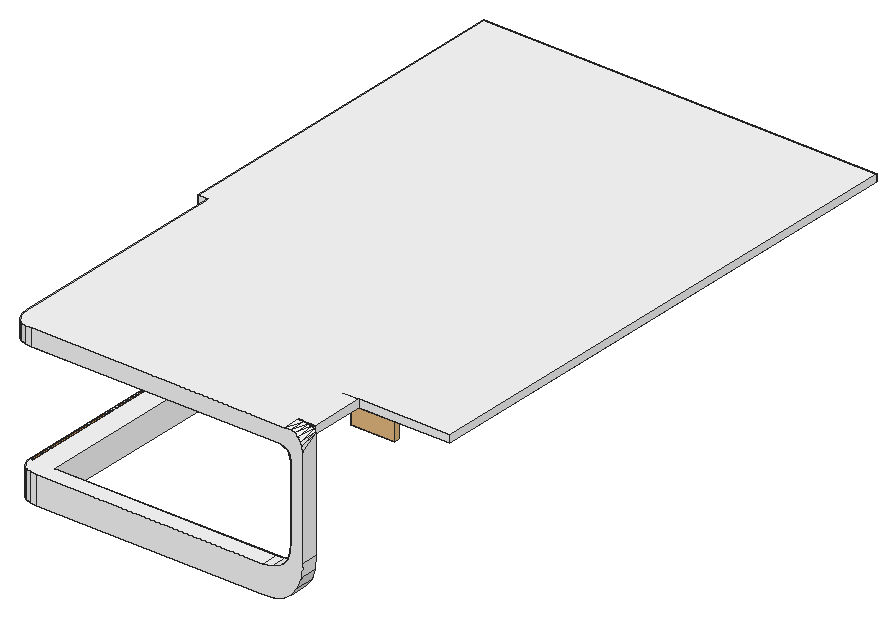
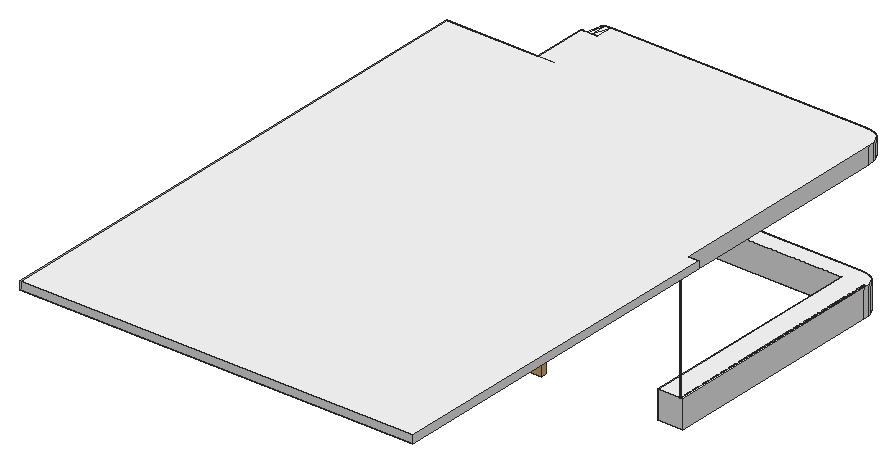
# SketchUp Ruby script. Lengths in inches.
U = 1.inch
M = Sketchup.active_model
def pt(a) = Geom::Point3d.new(a.map { |v| v * U })
def face(e, loops, mat)
  f = e.add_face(loops[0].map { |a| pt(a) })
  loops[1..].each { |l| e.add_face(l.map { |a| pt(a) }).erase! }
  f.material = f.back_material = mat if mat
  f
end
# faces: each face lists its corners as indices into pts; further lists are holes
def faces(e, pts, list, mat = nil) = list.each { |f| face(e, (f[0].is_a?(Array) ? f : [f]).map { |l| l.map { |i| pts[i] } }, mat) }
# xy, xz, yz: faces in a plane at the given z, y or x. An outline is a flat list of corners, or four numbers for a rectangle; further outlines are holes
def ring(l) = l.size == 4 ? [[l[0], l[1]], [l[2], l[1]], [l[2], l[3]], [l[0], l[3]]] : l.each_slice(2).to_a
def flat(e, list, mat, &to3) = list.each { |f| face(e, (f[0].is_a?(Array) ? f : [f]).map { |l| ring(l).map { |u, v| to3.(u, v) } }, mat) }
def xy(e, z, list, mat = nil) = flat(e, list, mat) { |x, y| [x, y, z] }
def xz(e, y, list, mat = nil) = flat(e, list, mat) { |x, z| [x, y, z] }
def yz(e, x, list, mat = nil) = flat(e, list, mat) { |y, z| [x, y, z] }
def lines(e, pts, list) = list.each { |a, b| e.add_line(pt(pts[a]), pt(pts[b])) }
# prism: a flat outline (further loops are holes) pulled along v
def prism(e, loops, v, mat = nil)
  f = face(e, loops, mat); d = Geom::Vector3d.new(v.map { |x| x * U })
  f.pushpull(f.normal.samedirection?(d) ? d.length : -d.length)
end
def box(e, o, s, mat = nil) = prism(e, [[o, [o[0] + s[0], o[1], o[2]], [o[0] + s[0], o[1] + s[1], o[2]], [o[0], o[1] + s[1], o[2]]]], [0, 0, s[2]], mat)
def at(x, y, z, deg = 0) = Geom::Transformation.translation(pt([x, y, z])) * Geom::Transformation.rotation(ORIGIN, Z_AXIS, deg.degrees)
def axes(o, x, y, z) = Geom::Transformation.new([*x, 0, *y, 0, *z, 0, *pt(o).to_a, 1])
def part(name) = M.definitions.add(name)
# library, detail: a bought-in or finely detailed component or shape, given as its bounding box
def library(name, o, s) = part(name).tap { |d| box(d.entities, o, s) }
def detail(e, o, s) = box(e.add_group.entities, o, s)
def put(e, d, t, mat = nil) = e.add_instance(d, t).tap { |i| i.material = mat if mat }
def group(e, t, mat = nil) = e.add_group.tap { |g| g.transformation = t; g.material = mat if mat }.entities
root = M.entities
M.materials.add("1056 AP 9903 Mellow Melon-N").color = [219, 142, 59]
M.materials.add("1117 AP 9945 Muted Auburn-N").color = [162, 88, 63]
M.materials.add("CTS CNC Default").color = [255, 255, 255]
c1 = library("Untitled",[0,0,0],[36,4.39,84])
c2 = part("Recessed ceiling light")
xy(c2.entities,-1,[[6,2,7.04,2.14,8,2.54,8.83,3.17,9.46,4,9.86,4.96,10,6,9.86,7.04,9.46,8,8.83,8.83,8,9.46,7.04,9.86,6,10,4.96,9.86,4,9.46,3.17,8.83,2.54,8,2.14,7.04,2,6,2.14,4.96,2.54,4,3.17,3.17,4,2.54,4.96,2.14]],"1117 AP 9945 Muted Auburn-N")
xy(c2.entities,0,[[[6,0,7.55,0.2,9,0.8,10.24,1.76,11.2,3,11.8,4.45,12,6,11.8,7.55,11.2,9,10.24,10.24,9,11.2,7.55,11.8,6,12,4.45,11.8,3,11.2,1.76,10.24,0.8,9,0.2,7.55,0,6,0.2,4.45,0.8,3,1.76,1.76,3,0.8,4.45,0.2],[6,2,4.96,2.14,4,2.54,3.17,3.17,2.54,4,2.14,4.96,2,6,2.14,7.04,2.54,8,3.17,8.83,4,9.46,4.96,9.86,6,10,7.04,9.86,8,9.46,8.83,8.83,9.46,8,9.86,7.04,10,6,9.86,4.96,9.46,4,8.83,3.17,8,2.54,7.04,2.14]]],"1117 AP 9945 Muted Auburn-N")
p = [[4.96,2.14,0],[6,2,0],[6,2,-1],[4.96,2.14,-1],[7.04,2.14,0],[7.04,2.14,-1],
  [4,2.54,0],[4,2.54,-1],[8,2.54,0],[8,2.54,-1],[3.17,3.17,0],[3.17,3.17,-1],
  [8.83,3.17,0],[8.83,3.17,-1],[2.54,4,0],[2.54,4,-1],[9.46,4,0],[9.46,4,-1],
  [2.14,4.96,0],[2.14,4.96,-1],[9.86,4.96,0],[9.86,4.96,-1],[2,6,0],[2,6,-1],
  [10,6,0],[10,6,-1],[2.14,7.04,0],[2.14,7.04,-1],[9.86,7.04,0],[9.86,7.04,-1],
  [2.54,8,0],[2.54,8,-1],[9.46,8,0],[9.46,8,-1],[3.17,8.83,0],[3.17,8.83,-1],
  [8.83,8.83,0],[8.83,8.83,-1],[4,9.46,0],[4,9.46,-1],[8,9.46,0],[8,9.46,-1],
  [4.96,9.86,0],[4.96,9.86,-1],[7.04,9.86,0],[7.04,9.86,-1],[6,10,0],[6,10,-1]]
faces(c2.entities,p,[[0,1,2,3],[1,4,5,2],[6,0,3,7],[4,8,9,5],[10,6,7,11],[8,12,13,9],[14,10,11,15],[12,16,17,13],
  [18,14,15,19],[16,20,21,17],[22,18,19,23],[20,24,25,21],[26,22,23,27],[24,28,29,25],[30,26,27,31],[28,32,33,29],
  [34,30,31,35],[32,36,37,33],[38,34,35,39],[36,40,41,37],[42,38,39,43],[40,44,45,41],[46,42,43,47],[44,46,47,45]],"1117 AP 9945 Muted Auburn-N")
xy(root,145.75,[[14.35,13.79,15.0625,202.3125]],"1056 AP 9903 Mellow Melon-N")
xz(root,202.3125,[[14.35,145.75,15.0625,238.4375]],"1056 AP 9903 Mellow Melon-N")
p = [[15.0625,202.3125,145.75],[15.0625,202.3125,238.4375],[15.0625,13.79,145.75]]
lines(root,p,[[0,1],[2,0]])
put(root,c1,at(123.5625,204.4,126))
g1 = group(root,at(21.875,58.1875,246),"CTS CNC Default")
xy(g1,-123,[[7.7,-58.1875,2.53,-57.72,-1.69,-56.31,-4.98,-53.96,-7.33,-50.67,-8.74,-46.45,-9.21,-41.28,-9.21,144.125,11.625,144.125,11.625,-44.375,191.93,-44.375,191.93,-58.1875]])
xy(g1,-100.25,[[7.7,-58.1875,193.39,-58.1875,193.39,-44.375,11.625,-44.375,11.625,144.125,-9.21,144.125,-9.21,-41.28,-8.74,-46.45,-7.33,-50.67,-4.98,-53.96,-1.69,-56.31,2.53,-57.72]])
xy(g1,-7.5625,[[4.05,-58.1875,-1.35,-57.7,-5.77,-56.22,-9.21,-53.77,-11.66,-50.33,-13.13,-45.91,-13.625,-40.51,-13.625,144.125,0,144.125,0,-44.375,205.85,-44.375,205.85,-58.1875]])
xy(g1,0,[[0,-44.375,0,144.125,300,144.125,300,0,225.17,0,225.17,-44.375]],"1117 AP 9945 Muted Auburn-N")
xy(g1,0,[[-21.875,144.125,300,436.5]],"CTS CNC Default")
xy(g1,6,[[4.05,-58.1875,211.44,-58.1875,211.44,-44.375,225.17,-44.375,225.17,0,300,0,300,436.5,-21.875,436.5,-21.875,144.125,-13.625,144.125,-13.625,-40.51,-13.13,-45.91,-11.66,-50.33,-9.21,-53.77,-5.77,-56.22,-1.35,-57.7]])
xz(g1,-58.1875,[[7.7,-123,191.93,-123,202.21,-122.07,210.62,-119.26,217.16,-114.59,221.83,-108.05,224.63,-99.65,225.5625,-89.37,225.5625,-7.5625,225.17,-3.42,223.99,-0.03,222.03,2.61,219.29,4.49,215.76,5.625,211.44,6,4.05,6,4.05,-7.5625,205.85,-7.5625,208.87,-7.84,211.33,-8.66,213.25,-10.03,214.625,-11.95,215.45,-14.42,215.72,-17.43,215.72,-77.91,215.1,-84.74,213.24,-90.32,210.14,-94.67,205.79,-97.77,200.21,-99.63,193.39,-100.25,7.7,-100.25]])
xz(g1,-44.375,[[11.625,-123,11.625,-100.25,193.39,-100.25,200.21,-99.63,205.79,-97.77,210.14,-94.67,213.24,-90.32,215.1,-84.74,215.72,-77.91,215.72,-17.43,215.45,-14.42,214.625,-11.95,213.25,-10.03,211.33,-8.66,208.87,-7.84,205.85,-7.5625,0,-7.5625,0,0,225.5625,0,225.5625,-89.37,224.63,-99.65,221.83,-108.05,217.16,-114.59,210.62,-119.26,202.21,-122.07,191.93,-123],[212.01,0,225.17,0,225.17,1.83,223.99,3.33,222.03,4.5,219.29,5.33,215.76,5.83,212.01,5.98],[225.17,0,225.5625,0,225.17,1.83],[225.17,1.83,225.17,5.98,212.01,5.98,215.76,5.83,219.29,5.33,222.03,4.5,223.99,3.33],[212.01,5.98,212.01,6,211.44,6],
  [212.01,5.98,225.17,6]])
xz(g1,0,[[225.17,0,300,6]])
xz(g1,144.125,[[-9.21,-123,11.625,-100.25],[-13.625,-7.5625,0,0],[-21.875,0,-13.625,6]])
xz(g1,436.5,[[-21.875,0,300,6]])
yz(g1,-21.875,[[144.125,0,436.5,6]])
yz(g1,-13.625,[[-40.51,-7.5625,144.125,6]])
yz(g1,-9.21,[[-41.28,-123,144.125,-100.25]])
yz(g1,0,[[-44.375,-7.5625,144.125,0]])
yz(g1,11.625,[[-44.375,-123,144.125,-100.25]])
yz(g1,215.72,[[-58.1875,-77.91,-44.375,-17.43]])
yz(g1,225.17,[[-44.375,0,0,6]])
yz(g1,225.5625,[[-58.1875,-89.37,-44.375,-89.37,-44.375,0,-58.1875,-7.5625]])
yz(g1,300,[[0,0,436.5,6]])
p = [[2.53,-57.72,-100.25],[2.53,-57.72,-123],[7.7,-58.1875,-123],[7.7,-58.1875,-100.25],[202.21,-44.375,-122.07],[202.21,-58.1875,-122.07],
  [191.93,-58.1875,-123],[191.93,-44.375,-123],[-1.69,-56.31,-100.25],[-1.69,-56.31,-123],[-4.98,-53.96,-100.25],[-4.98,-53.96,-123],
  [-7.33,-50.67,-100.25],[-7.33,-50.67,-123],[-8.74,-46.45,-100.25],[-8.74,-46.45,-123],[-9.21,-41.28,-100.25],[-9.21,-41.28,-123],
  [210.62,-44.375,-119.26],[210.62,-58.1875,-119.26],[217.16,-44.375,-114.59],[217.16,-58.1875,-114.59],[221.83,-44.375,-108.05],[221.83,-58.1875,-108.05],
  [224.63,-44.375,-99.65],[224.63,-58.1875,-99.65],[193.39,-44.375,-100.25],[193.39,-58.1875,-100.25],[200.21,-58.1875,-99.63],[200.21,-44.375,-99.63],
  [205.79,-58.1875,-97.77],[205.79,-44.375,-97.77],[225.5625,-44.375,-89.37],[225.5625,-58.1875,-89.37],[210.14,-58.1875,-94.67],[210.14,-44.375,-94.67],
  [213.24,-58.1875,-90.32],[213.24,-44.375,-90.32],[215.1,-58.1875,-84.74],[215.1,-44.375,-84.74],[215.72,-58.1875,-77.91],[215.72,-44.375,-77.91],
  [215.72,-44.375,-17.43],[215.72,-58.1875,-17.43],[215.45,-58.1875,-14.42],[215.45,-44.375,-14.42],[214.625,-58.1875,-11.95],[214.625,-44.375,-11.95],
  [213.25,-58.1875,-10.03],[213.25,-44.375,-10.03],[211.33,-58.1875,-8.66],[211.33,-44.375,-8.66],[208.87,-58.1875,-7.84],[208.87,-44.375,-7.84],
  [205.85,-58.1875,-7.5625],[205.85,-44.375,-7.5625],[-1.35,-57.7,6],[-1.35,-57.7,-7.5625],[4.05,-58.1875,-7.5625],[4.05,-58.1875,6],
  [225.5625,-58.1875,-7.5625],[225.5625,-44.375,0],[225.17,-58.1875,-3.42],[-5.77,-56.22,6],[-5.77,-56.22,-7.5625],[-9.21,-53.77,6],
  [-9.21,-53.77,-7.5625],[-11.66,-50.33,6],[-11.66,-50.33,-7.5625],[-13.13,-45.91,6],[-13.13,-45.91,-7.5625],[-13.625,-40.51,6],
  [-13.625,-40.51,-7.5625],[225.17,-44.375,1.83],[223.99,-58.1875,-0.03],[223.99,-44.375,3.33],[222.03,-58.1875,2.61],[222.03,-44.375,4.5],
  [219.29,-58.1875,4.49],[219.29,-44.375,5.33],[215.76,-58.1875,5.625],[215.76,-44.375,5.83],[211.44,-58.1875,6],[212.01,-44.375,5.98],
  [211.44,-44.375,6],[225.17,0,6],[212.01,0,6],[212.01,0,0]]
faces(g1,p,[[0,1,2,3],[4,5,6,7],[8,9,1,0],[10,11,9,8],[12,13,11,10],[14,15,13,12],[16,17,15,14],[18,19,5,4],
  [20,21,19,18],[22,23,21,20],[24,25,23,22],[26,27,28,29],[29,28,30,31],[32,33,25,24],[31,30,34,35],[35,34,36,37],
  [37,36,38,39],[39,38,40,41],[42,43,44,45],[45,44,46,47],[47,46,48,49],[49,48,50,51],[51,50,52,53],[53,52,54,55],
  [56,57,58,59],[60,61,62],[63,64,57,56],[65,66,64,63],[67,68,66,65],[69,70,68,67],[71,72,70,69],[62,73,74],
  [61,73,62],[74,75,76],[73,75,74],[76,77,78],[75,77,76],[78,79,80],[77,79,78],[79,81,80],
  [80,81,82],[83,84,82,81]])
lines(g1,p,[[85,86],[87,86]])
put(g1,c2,axes([23.23,-30.51,0],[-1,0,0],[0,1,0],[0,0,-1]))
put(g1,c2,axes([86.8,-30.51,0],[-1,0,0],[0,1,0],[0,0,-1]))
put(g1,c2,axes([150.37,-30.51,0],[-1,0,0],[0,1,0],[0,0,-1]))
put(g1,c2,axes([213.9375,-30.51,0],[-1,0,0],[0,1,0],[0,0,-1]))
put(g1,c2,axes([86.8,121.89,0],[-1,0,0],[0,1,0],[0,0,-1]))
put(g1,c2,axes([213.9375,121.89,0],[-1,0,0],[0,1,0],[0,0,-1]))
put(g1,c2,axes([150.37,121.89,0],[-1,0,0],[0,1,0],[0,0,-1]))
put(g1,c2,axes([23.23,121.89,0],[-1,0,0],[0,1,0],[0,0,-1]))
put(g1,c2,axes([86.8,20.29,0],[-1,0,0],[0,1,0],[0,0,-1]))
put(g1,c2,axes([213.9375,20.29,0],[-1,0,0],[0,1,0],[0,0,-1]))
put(g1,c2,axes([150.37,20.29,0],[-1,0,0],[0,1,0],[0,0,-1]))
put(g1,c2,axes([23.23,20.29,0],[-1,0,0],[0,1,0],[0,0,-1]))
put(g1,c2,axes([86.8,71.09,0],[-1,0,0],[0,1,0],[0,0,-1]))
put(g1,c2,axes([213.9375,71.09,0],[-1,0,0],[0,1,0],[0,0,-1]))
put(g1,c2,axes([150.37,71.09,0],[-1,0,0],[0,1,0],[0,0,-1]))
put(g1,c2,axes([23.23,71.09,0],[-1,0,0],[0,1,0],[0,0,-1]))
put(g1,c2,axes([86.8,121.89,0],[-1,0,0],[0,1,0],[0,0,-1]))
put(g1,c2,axes([213.9375,121.89,0],[-1,0,0],[0,1,0],[0,0,-1]))
put(g1,c2,axes([150.37,121.89,0],[-1,0,0],[0,1,0],[0,0,-1]))
put(g1,c2,axes([23.23,121.89,0],[-1,0,0],[0,1,0],[0,0,-1]))
